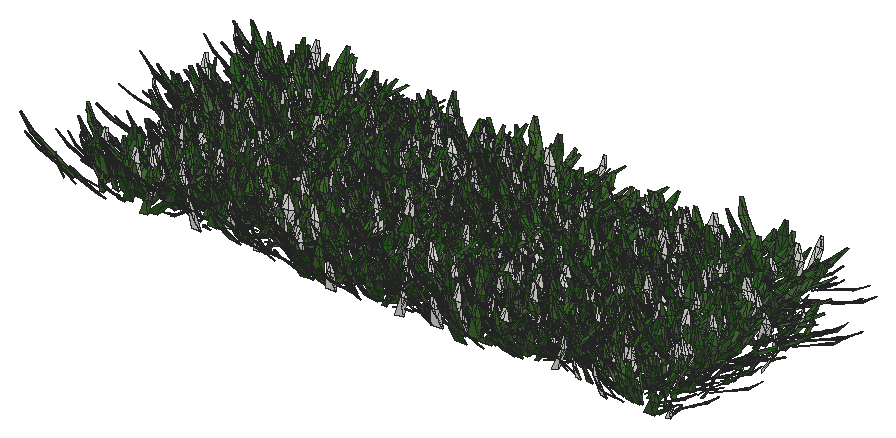
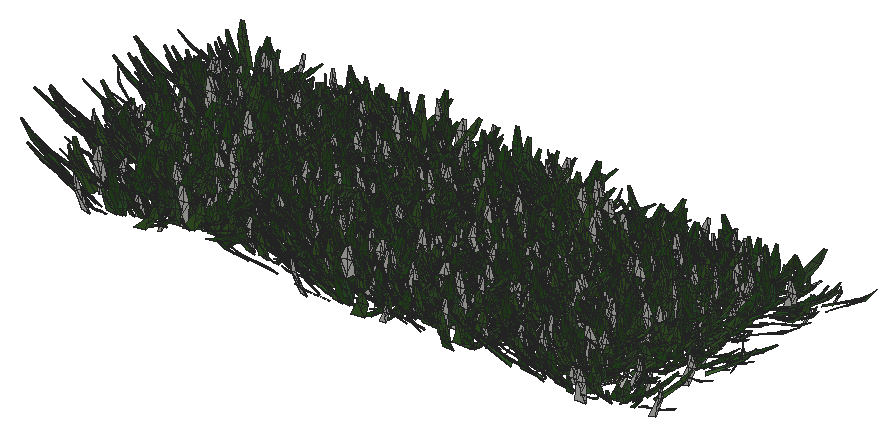
# SketchUp Ruby script. Lengths in inches.
U = 1.inch
M = Sketchup.active_model
def pt(a) = Geom::Point3d.new(a.map { |v| v * U })
def face(e, loops, mat)
  f = e.add_face(loops[0].map { |a| pt(a) })
  loops[1..].each { |l| e.add_face(l.map { |a| pt(a) }).erase! }
  f.material = f.back_material = mat if mat
  f
end
# faces: each face lists its corners as indices into pts; further lists are holes
def faces(e, pts, list, mat = nil) = list.each { |f| face(e, (f[0].is_a?(Array) ? f : [f]).map { |l| l.map { |i| pts[i] } }, mat) }
# xy, xz, yz: faces in a plane at the given z, y or x. An outline is a flat list of corners, or four numbers for a rectangle; further outlines are holes
def ring(l) = l.size == 4 ? [[l[0], l[1]], [l[2], l[1]], [l[2], l[3]], [l[0], l[3]]] : l.each_slice(2).to_a
def flat(e, list, mat, &to3) = list.each { |f| face(e, (f[0].is_a?(Array) ? f : [f]).map { |l| ring(l).map { |u, v| to3.(u, v) } }, mat) }
def xy(e, z, list, mat = nil) = flat(e, list, mat) { |x, y| [x, y, z] }
def xz(e, y, list, mat = nil) = flat(e, list, mat) { |x, z| [x, y, z] }
def yz(e, x, list, mat = nil) = flat(e, list, mat) { |y, z| [x, y, z] }
def lines(e, pts, list) = list.each { |a, b| e.add_line(pt(pts[a]), pt(pts[b])) }
# prism: a flat outline (further loops are holes) pulled along v
def prism(e, loops, v, mat = nil)
  f = face(e, loops, mat); d = Geom::Vector3d.new(v.map { |x| x * U })
  f.pushpull(f.normal.samedirection?(d) ? d.length : -d.length)
end
def box(e, o, s, mat = nil) = prism(e, [[o, [o[0] + s[0], o[1], o[2]], [o[0] + s[0], o[1] + s[1], o[2]], [o[0], o[1] + s[1], o[2]]]], [0, 0, s[2]], mat)
def at(x, y, z, deg = 0) = Geom::Transformation.translation(pt([x, y, z])) * Geom::Transformation.rotation(ORIGIN, Z_AXIS, deg.degrees)
def axes(o, x, y, z) = Geom::Transformation.new([*x, 0, *y, 0, *z, 0, *pt(o).to_a, 1])
def part(name) = M.definitions.add(name)
# library, detail: a bought-in or finely detailed component or shape, given as its bounding box
def library(name, o, s) = part(name).tap { |d| box(d.entities, o, s) }
def detail(e, o, s) = box(e.add_group.entities, o, s)
def put(e, d, t, mat = nil) = e.add_instance(d, t).tap { |i| i.material = mat if mat }
def group(e, t, mat = nil) = e.add_group.tap { |g| g.transformation = t; g.material = mat if mat }.entities
root = M.entities
M.materials.add("Material82").color = [68, 110, 58]
M.materials.add("Material83").color = [48, 90, 38]
M.materials.add("Material84").color = [68, 110, 48]
M.materials.add("Material85").color = [48, 90, 48]
M.materials.add("Material86").color = [58, 110, 58]
M.materials.add("Material87").color = [58, 90, 38]
M.materials.add("Material88").color = [68, 100, 58]
M.materials.add("Material89").color = [48, 100, 38]
c1 = part("grass00")
p = [[-0.6875,0.15,0],[-0.56,0.08,5.52],[-0.04,0.03,2.76],[0.48,-0.02,0],[0.35,-0.02,5.52],[-0.1,-0.14,5.52],
  [-0.12,0.65,8.37],[-0.42,0.65,8.37]]
faces(c1.entities,p,[[0,1,2,3],[3,2,4],[1,5,2],[5,4,2],[1,6,5],[4,5,6],[7,6,1]])
c2 = part("Group16\#1")
put(c2.entities,c1,axes([1.44,-0.61,-0.01],[0.05352,0.12609,0],[-0.10704,0.04543,0.07239],[0.06664,-0.02828,0.11628]),"Material85")
put(c2.entities,c1,axes([0.76,-0.15,-0.01],[0.04676,0.24062,0],[-0.23162,0.04501,0.06642],[0.0652,-0.01267,0.23595]),"Material82")
put(c2.entities,c1,axes([0.79,0.01,-0.01],[-0.00606,0.34651,0],[-0.34381,-0.00602,0.0432],[0.04319,0.00076,0.34386]))
put(c2.entities,c1,axes([1,0.23,-0.01],[-0.07192,0.31144,0],[-0.28722,-0.06632,0.1236],[0.12043,0.02781,0.29478]),"Material84")
put(c2.entities,c1,axes([1.66,0.77,-0.01],[-0.13828,0.29651,0],[-0.21551,-0.1005,0.22471],[0.20365,0.09498,0.23779]),"Material89")
put(c2.entities,c1,axes([0.6875,0.52,-0.01],[-0.18126,0.24051,0],[-0.22746,-0.17142,0.09788],[0.07817,0.05891,0.28481]),"Material84")
put(c2.entities,c1,axes([0.68,0.78,-0.01],[-0.215,0.18688,0],[-0.12385,-0.14248,0.21334],[0.13995,0.16101,0.18878]),"Material82")
put(c2.entities,c1,axes([0.56,1,-0.01],[-0.13756,0.07624,0],[-0.06159,-0.11112,0.0927],[0.04494,0.08108,0.12705]),"Material84")
put(c2.entities,c1,axes([0.2,0.64,-0.01],[-0.23729,0.07254,0],[-0.05711,-0.18681,0.153],[0.04473,0.14632,0.19535]),"Material89")
put(c2.entities,c1,axes([0.0625,0.72,-0.01],[-0.28874,0.02525,0],[-0.02179,-0.24916,0.14647],[0.01276,0.14591,0.25012]),"Material82")
put(c2.entities,c1,axes([-0.08,0.62,-0.01],[-0.34089,-0.04187,0],[0.03255,-0.26504,0.216],[-0.02633,0.21439,0.26703]),"Material89")
put(c2.entities,c1,axes([-0.34,0.98,-0.01],[-0.14314,-0.0493,0],[0.04397,-0.12769,0.06843],[-0.02228,0.0647,0.13505]),"Material89")
put(c2.entities,c1,axes([-0.87,1.45,-0.01],[-0.23488,-0.14114,0],[0.13761,-0.22901,0.06087],[-0.03135,0.05217,0.26717]))
put(c2.entities,c1,axes([-0.72,0.77,-0.01],[-0.14208,-0.13251,0],[0.07209,-0.0773,0.16301],[-0.11118,0.11922,0.1057]),"Material89")
put(c2.entities,c1,axes([-0.62,0.43,-0.01],[-0.14845,-0.21203,0],[0.18654,-0.13061,0.12304],[-0.10079,0.07057,0.22772]),"Material82")
put(c2.entities,c1,axes([-0.68,0.29,-0.01],[-0.13639,-0.32136,0],[0.31723,-0.13464,0.05579],[-0.05136,0.0218,0.34462]),"Material83")
put(c2.entities,c1,axes([-0.64,0.125,-0.01],[-0.0458,-0.23569,0],[0.22124,-0.043,0.08276],[-0.08124,0.01579,0.22538]),"Material86")
put(c2.entities,c1,axes([-1.6,-0.03,-0.01],[0.00576,-0.32897,0],[0.27526,0.00482,0.18018],[-0.18015,-0.00315,0.2753]),"Material84")
put(c2.entities,c1,axes([-1.36,-0.31,-0.01],[0.05718,-0.24765,0],[0.18172,0.04196,0.17267],[-0.16825,-0.03885,0.1865]),"Material89")
put(c2.entities,c1,axes([-1.54,-0.72,-0.01],[0.06537,-0.14017,0],[0.13555,0.06321,0.03939],[-0.0357,-0.01665,0.14956]))
put(c2.entities,c1,axes([-1.19,-0.9,-0.01],[0.09597,-0.12735,0],[0.11214,0.08451,0.07557],[-0.06035,-0.04548,0.14042]),"Material88")
put(c2.entities,c1,axes([-0.47,-0.54,-0.01],[0.11588,-0.10072,0],[0.0618,0.0711,0.12124],[-0.07953,-0.0915,0.0942]))
put(c2.entities,c1,axes([-0.47,-0.84,-0.01],[0.11927,-0.0661,0],[0.06603,0.11913,0.00646],[-0.00313,-0.00565,0.13621]),"Material84")
put(c2.entities,c1,axes([-0.38,-1.24,-0.01],[0.28037,-0.08571,0],[0.0618,0.20215,0.20315],[-0.05939,-0.19428,0.21139]),"Material88")
put(c2.entities,c1,axes([-0.06,-0.66,-0.01],[0.22719,-0.01987,0],[0.01247,0.14255,0.17758],[-0.01547,-0.17691,0.1431]),"Material87")
put(c2.entities,c1,axes([0.11,-0.89,-0.01],[0.14882,0.01828,0],[-0.01058,0.08611,0.12229],[0.01491,-0.12138,0.08676]),"Material85")
put(c2.entities,c1,axes([0.25,-0.72,-0.01],[0.20481,0.07053,0],[-0.06206,0.18022,0.10291],[0.03351,-0.0973,0.1906]),"Material85")
put(c2.entities,c1,axes([0.85,-1.42,-0.01],[0.16481,0.09904,0],[-0.09472,0.15762,0.05616],[0.02893,-0.04814,0.18389]),"Material84")
put(c2.entities,c1,axes([1.01,-1.09,-0.01],[0.21858,0.20385,0],[-0.17495,0.1876,0.15339],[0.10462,-0.11218,0.25652]),"Material89")
put(c2.entities,c1,axes([1.01,-0.71,-0.01],[0.08733,0.12473,0],[-0.06445,0.04512,0.13037],[0.1068,-0.07477,0.07867]),"Material85")
c3 = part("Group15\#1")
put(c3.entities,c2,at(0,0,0))
c4 = part("3darcstudiotree_grass00\#1")
put(c4.entities,c3,at(0,0,0))
put(root,c4,axes([1821.52,342.86,-34.17],[3.14963,-1.20842,0],[2.29792,0.93151,-0.01443],[0.07601,0.03081,1.86565]))
put(root,c4,axes([1822.68,356.8,-34.17],[-4.00454,-0.52801,0],[1.05814,-1.24816,-0.00172],[0.00311,-0.00367,1.42531]))
put(root,c4,axes([1822.78,343.67,-34.17],[-1.0046,-1.54951,0],[3.94346,-0.39764,-0.04783],[0.24428,-0.02463,1.6084]))
put(root,c4,axes([1821.28,366.74,-34.17],[2.75664,0.78459,0],[-2.60411,1.42301,-0.01696],[-0.0547,0.02989,1.8379]))
put(root,c4,axes([1821.49,355.92,-34.17],[1.57656,1.15501,0],[-3.7913,0.80487,-0.00648],[-0.02974,0.00631,1.68262]))
put(root,c4,axes([1823.79,345.66,-34.17],[-0.37683,-1.42813,0],[4.6236,-0.18974,-0.00351],[0.01488,-0.00061,1.48465]))
put(root,c4,axes([1822,340.73,-34.17],[4.54007,0.12562,0],[-0.30482,1.71344,-0.05051],[-0.02069,0.11631,1.91076]))
put(root,c4,axes([1823.4,350.05,-34.17],[1.62707,-1.18617,0],[3.8873,0.82932,-0.03985],[0.15889,0.0339,1.5017]))
put(root,c4,axes([1822.96,359.32,-34.17],[4.17569,0.70475,0],[-1.86329,1.71705,-0.06274],[-0.13365,0.12316,1.92197]))
put(root,c4,axes([1825.36,351.61,-34.17],[-3.80347,-0.79702,0],[1.88494,-1.39901,-0.03648],[0.10192,-0.07565,1.79293]))
put(root,c4,axes([1825.29,349.31,-34.17],[-2.17021,-1.46243,0],[2.84473,-0.65657,-0.0221],[0.14072,-0.03248,1.82262]))
put(root,c4,axes([1826.87,353.74,-34.17],[-2.18591,-1.17845,0],[3.11783,-0.89946,-0.02018],[0.10185,-0.02938,1.81061]))
put(root,c4,axes([1825.55,367.79,-34.17],[4.09864,-0.14348,0],[0.37168,1.65134,-0.01913],[0.00999,0.04439,1.86132]))
put(root,c4,axes([1826.16,355.56,-34.17],[-1.78032,1.61918,0],[-3.86174,-0.66038,-0.00354],[-0.01693,-0.0029,1.64409]))
put(root,c4,axes([1827.11,342.72,-34.17],[3.03313,0.50579,0],[-1.37798,1.28522,-0.04149],[-0.11611,0.10829,1.90578]))
put(root,c4,axes([1827.04,343.85,-34.17],[4.0409,0.57443,0],[-1.45336,1.59011,-0.05978],[-0.09434,0.10321,1.49495]))
put(root,c4,axes([1826.91,364.67,-34.17],[3.09052,1.16305,0],[-2.75216,1.13741,-0.00767],[-0.03246,0.01341,1.8325]))
put(root,c4,axes([1828.08,346.72,-34.17],[1.55138,-1.30688,0],[2.99369,0.55272,-0.04141],[0.29892,0.05519,1.97468]))
put(root,c4,axes([1827.93,360.0625,-34.17],[4.14328,-0.46419,0],[1.00154,1.39037,-0.02465],[0.03463,0.04808,1.41248]))
put(root,c4,axes([1828.45,358.2,-34.17],[-0.77153,1.33479,0],[-3.28421,-0.29525,-0.03421],[-0.24787,-0.02228,1.87625]))
put(root,c4,axes([1828.79,361.74,-34.17],[-1.91367,1.54924,0],[-4.25661,-0.81775,-0.00711],[-0.02422,-0.00465,1.34501]))
put(root,c4,axes([1829.4,366.36,-34.17],[3.43874,0.27286,0],[-0.6732,1.31953,-0.0192],[-0.02432,0.04768,1.64321]))
put(root,c4,axes([1830.92,343.8125,-34.17],[-4.1133,-0.05921,0],[0.15009,-1.6218,-0.04384],[0.00865,-0.09349,1.66887]))
put(root,c4,axes([1831.73,341.69,-34.17],[-3.5543,0.89209,0],[-1.79933,-1.11498,-0.04609],[-0.16829,-0.10428,1.7083]))
put(root,c4,axes([1832.4375,346.45,-34.17],[-2.34222,-1.01748,0],[3.28821,-1.17726,-0.05879],[0.21723,-0.07777,1.66118]))
put(root,c4,axes([1831.48,363.76,-34.17],[3.65348,-0.50094,0],[1.24961,1.41744,-0.02118],[0.04225,0.04793,1.73224]))
put(root,c4,axes([1832.65,359.43,-34.17],[-0.28709,-1.61704,0],[4.14071,-0.11434,-0.04142],[0.22933,-0.00633,1.72685]))
put(root,c4,axes([1831.33,366.19,-34.17],[1.27855,1.29921,0],[-4.02019,0.61532,-0.04732],[-0.19364,0.02964,1.41896]))
put(root,c4,axes([1831.85,350.0625,-34.17],[-1.96915,1.54328,0],[-4.06414,-0.80652,-0.00338],[-0.01619,-0.00321,1.82725]))
put(root,c4,axes([1833.39,349.04,-34.17],[-3.56597,0.54096,0],[-1.21057,-1.24113,-0.01112],[-0.02689,-0.02757,1.70172]))
put(root,c4,axes([1832.2,361.6,-34.17],[3.55843,0.77732,0],[-2.07504,1.47739,-0.02111],[-0.0608,0.04329,1.90804]))
put(root,c4,axes([1832.72,357.15,-34.17],[4.24476,0.21314,0],[-0.43337,1.34235,-0.04636],[-0.04216,0.1306,1.85211]))
put(root,c4,axes([1834.71,354.75,-34.17],[-3.8899,-0.78174,0],[2.11548,-1.63718,-0.02171],[0.04442,-0.03438,1.57387]))
put(root,c4,axes([1834.73,353.11,-34.17],[3.28347,0.12106,0],[-0.38901,1.64106,-0.04931],[-0.02254,0.09507,1.538]))
put(root,c4,axes([1837.52,354.72,-34.17],[-3.55041,0.9087,0],[-2.02381,-1.22981,-0.02727],[-0.0752,-0.0457,1.41127]))
put(root,c4,axes([1837.07,359.69,-34.17],[1.12356,1.5327,0],[-3.46853,0.39546,-0.04889],[-0.25471,0.02904,1.46761]))
put(root,c4,axes([1838.625,344.57,-34.17],[1.64327,-1.14246,0],[4.09949,0.91708,-0.03953],[0.17253,0.0386,1.77239]))
put(root,c4,axes([1837.41,342.6,-34.17],[0.41174,1.83159,0],[-3.96576,0.13865,-0.0152],[-0.08151,0.00285,1.60635]))
put(root,c4,axes([1839.55,348.04,-34.17],[0.23576,-1.73441,0],[4.70751,0.09952,-0.00697],[0.03732,0.00079,1.89407]))
put(root,c4,axes([1839.34,352.72,-34.17],[-3.49986,-0.57002,0],[1.44663,-1.38143,-0.04671],[0.11633,-0.11108,1.85324]))
put(root,c4,axes([1838.43,346.12,-34.17],[0.9145,1.75116,0],[-3.69114,0.2998,-0.03105],[-0.20233,0.01643,1.87912]))
put(root,c4,axes([1838.69,350.85,-34.17],[1.28043,1.73979,0],[-3.30316,0.37809,-0.03743],[-0.19576,0.02241,1.40382]))
put(root,c4,axes([1839.18,361.54,-34.17],[2.41483,0.92576,0],[-3.06998,1.24547,-0.04673],[-0.14351,0.05822,1.45453]))
put(root,c4,axes([1839.63,363.54,-34.17],[4.28624,-0.48224,0],[1.29741,1.79351,-0.04256],[0.05122,0.07081,1.55488]))
put(root,c4,axes([1839.96,365.39,-34.17],[0.63995,1.63517,0],[-3.50377,0.21327,-0.04631],[-0.28502,0.01735,1.65491]))
put(root,c4,axes([1840.43,357.61,-34.17],[4.08655,-0.74198,0],[1.4526,1.2443,-0.00355],[0.00912,0.00781,1.60125]))
put(root,c4,axes([1840.41,367.56,-34.17],[1.05791,1.29898,0],[-3.4169,0.4328,-0.04361],[-0.24845,0.03147,1.60948]))
put(root,c4,axes([1842.04,355.39,-34.17],[-0.24051,-1.38856,0],[3.98568,-0.10737,-0.04502],[0.19517,-0.00526,1.30109]))
put(root,c4,axes([1843.08,344.86,-34.17],[1.00632,-1.60929,0],[3.83281,0.37276,-0.00763],[0.0458,0.00445,1.82848]))
put(root,c4,axes([1843.68,350.2,-34.17],[-2.49579,-0.85332,0],[2.16334,-0.98408,-0.00893],[0.04692,-0.02134,1.98619]))
put(root,c4,axes([1843.63,364.02,-34.17],[2.15184,-1.02148,0],[3.44742,1.1295,-0.00974],[0.03611,0.01183,1.619]))
put(root,c4,axes([1844,352.47,-34.17],[-3.56783,-0.13568,0],[0.42403,-1.73414,-0.0118],[0.00459,-0.01877,1.34216]))
put(root,c4,axes([1843.34,357,-34.17],[4.22834,-0.67564,0],[1.61938,1.57623,-0.01357],[0.03127,0.03043,1.98263]))
put(root,c4,axes([1843.62,346.92,-34.17],[3.42011,0.99957,0],[-2.24279,1.19352,-0.03152],[-0.09807,0.05219,1.47514]))
put(root,c4,axes([1845.72,341.58,-34.17],[-0.92987,-1.7368,0],[3.78348,-0.31505,-0.00703],[0.03581,-0.00298,1.50812]))
put(root,c4,axes([1844.32,358.77,-34.17],[3.74003,-0.3626,0],[0.86697,1.39078,-0.02888],[0.04393,0.07047,1.73467]))
put(root,c4,axes([1845.92,349.15,-34.17],[-2.16285,-1.07783,0],[3.1191,-0.97346,-0.00813],[0.02825,-0.00882,1.32168]))
put(root,c4,axes([1844.33,366.05,-34.17],[2.54513,1.12368,0],[-2.54126,0.89522,-0.01423],[-0.07597,0.02676,1.82816]))
put(root,c4,axes([1845.34,362.52,-34.17],[-2.35271,1.42324,0],[-3.1761,-0.81658,-0.00573],[-0.02769,-0.00712,1.63969]))
put(root,c4,axes([1847.43,362.21,-34.17],[-2.99545,-1.01525,0],[2.44315,-1.12112,-0.00129],[0.00439,-0.00201,1.46122]))
put(root,c4,axes([1847.8,340.5,-34.17],[-4.11359,0.33172,0],[-0.73599,-1.4195,-0.0347],[-0.04072,-0.07853,1.61275]))
put(root,c4,axes([1849.05,355.09,-34.17],[-1.26006,-1.32624,0],[4.43512,-0.65537,-0.00645],[0.02239,-0.00331,1.31612]))
put(root,c4,axes([1847.46,347.21,-34.17],[0.26665,1.72733,0],[-3.78087,0.09078,-0.02381],[-0.14887,0.00357,1.77807]))
put(root,c4,axes([1848.7,356.875,-34.17],[0.22416,-1.4452,0],[4.13727,0.09981,-0.05271],[0.23324,0.00563,1.37729]))
put(root,c4,axes([1848.47,341.31,-34.17],[2.00643,-1.16557,0],[2.7626,0.73963,-0.03969],[0.18592,0.04978,1.41714]))
put(root,c4,axes([1849.375,353.65,-34.17],[-2.85144,-1.16634,0],[2.50888,-0.95396,-0.03577],[0.14723,-0.05598,1.49339]))
put(root,c4,axes([1848.15,350.85,-34.17],[1.02208,1.31259,0],[-4.10151,0.49672,-0.03259],[-0.17155,0.02078,1.77089]))
put(root,c4,axes([1848.15,364.71,-34.17],[2.93363,1.22701,0],[-2.56818,0.95498,-0.02839],[-0.14721,0.05474,1.88589]))
put(root,c4,axes([1850.06,360.3,-34.17],[-0.17296,-1.31916,0],[4.52056,-0.09218,-0.00424],[0.01978,-0.0004,1.58408]))
put(root,c4,axes([1851.19,348.625,-34.17],[-4.36692,-0.69342,0],[1.6396,-1.60594,-0.01703],[0.03175,-0.0311,1.64249]))
put(root,c4,axes([1851.2,365.94,-34.17],[-4.04807,0.23611,0],[-0.60438,-1.61163,-0.04443],[-0.03837,-0.10233,1.82802]))
put(root,c4,axes([1849.74,344.16,-34.17],[3.28108,0.9921,0],[-2.06723,1.06332,-0.03117],[-0.09708,0.04994,1.30357]))
put(root,c4,axes([1853.22,360.25,-34.17],[-3.17197,-0.90891,0],[2.49685,-1.35522,-0.03763],[0.13517,-0.07337,1.94544]))
put(root,c4,axes([1853.55,351.03,-34.17],[-3.35579,-1.19548,0],[2.90415,-1.2679,-0.0585],[0.2305,-0.10063,1.90866]))
put(root,c4,axes([1853.41,368.26,-34.17],[1.68348,-1.42,0],[3.90393,0.71983,-0.01397],[0.0682,0.01258,1.74087]))
put(root,c4,axes([1852.96,358.17,-34.17],[-1.26035,1.30994,0],[-3.37363,-0.50484,-0.03389],[-0.19382,-0.029,1.65454]))
put(root,c4,axes([1854.15,340.4,-34.17],[-3.39608,-0.38473,0],[1.21289,-1.66516,-0.05258],[0.08123,-0.11153,1.84274]))
put(root,c4,axes([1854.58,347.85,-34.17],[-0.07574,-1.47303,0],[4.38332,-0.03505,-0.05384],[0.21677,-0.00173,1.32332]))
put(root,c4,axes([1854.56,352.84,-34.17],[-3.58969,-0.07657,0],[0.18796,-1.37056,-0.00522],[0.00152,-0.01105,1.40302]))
put(root,c4,axes([1854.63,364.52,-34.17],[-3.78052,0.58265,0],[-1.19847,-1.20943,-0.02866],[-0.07958,-0.08031,1.88291]))
put(root,c4,axes([1855.4,355.84,-34.17],[-3.3619,-0.88005,0],[2.60897,-1.55009,-0.03911],[0.08798,-0.05227,1.43856]))
put(root,c4,axes([1854.84,345.96,-34.17],[-0.00326,-1.3732,0],[3.39922,-0.00125,-0.0371],[0.2688,-0.0001,1.84609]))
put(root,c4,axes([1855.62,365.9,-34.17],[-2.81078,-0.75848,0],[2.18011,-1.25652,-0.01797],[0.04803,-0.02768,1.36964]))
put(root,c4,axes([1854.7,344.97,-34.17],[3.61578,-1.02121,0],[2.66994,1.47029,-0.04389],[0.14306,0.07878,1.92393]))
put(root,c4,axes([1855.75,342.71,-34.17],[3.76801,-0.42175,0],[1.14915,1.59678,-0.03157],[0.04846,0.06733,1.77323]))
put(root,c4,axes([1856.05,361.52,-34.17],[2.09185,1.03032,0],[-2.8732,0.90727,-0.01526],[-0.08429,0.02662,1.9517]))
put(root,c4,axes([1859.09,351.16,-34.17],[-1.37112,-1.31689,0],[3.73876,-0.60543,-0.04381],[0.2334,-0.0378,1.74465]))
put(root,c4,axes([1859.71,364.17,-34.17],[-0.8424,-1.2576,0],[4.34376,-0.45254,-0.01354],[0.07406,-0.00772,1.90468]))
put(root,c4,axes([1858.9,358.94,-34.17],[3.65327,1.04493,0],[-2.10749,1.14596,-0.01189],[-0.03901,0.02121,1.50367]))
put(root,c4,axes([1860.14,354.6,-34.17],[-2.51613,1.14478,0],[-2.79457,-0.95529,-0.04719],[-0.16752,-0.05727,1.30223]))
put(root,c4,axes([1859.1875,365.96,-34.17],[3.43468,1.02641,0],[-2.59272,1.34938,-0.0181],[-0.04577,0.02382,1.34745]))
put(root,c4,axes([1860.95,341.85,-34.17],[-4.19905,0.34301,0],[-0.96105,-1.82979,-0.05761],[-0.05651,-0.10759,1.71741]))
put(root,c4,axes([1860.14,362.37,-34.17],[3.21656,-1.06764,0],[2.25071,1.05463,-0.04982],[0.17505,0.08203,1.4295]))
put(root,c4,axes([1861.58,345.05,-34.17],[0.12061,-1.58998,0],[4.18389,0.04936,-0.01737],[0.08566,0.00101,1.54781]))
put(root,c4,axes([1862.15,356.91,-34.17],[-3.70247,-0.49757,0],[1.50858,-1.74588,-0.06303],[0.09341,-0.1081,1.61067]))
put(root,c4,axes([1861.14,347.21,-34.17],[-0.34365,1.56469,0],[-3.45908,-0.11816,-0.04948],[-0.26965,-0.00921,1.42361]))
put(root,c4,axes([1860.69,352.77,-34.17],[1.76415,1.1719,0],[-3.51067,0.82196,-0.05173],[-0.20066,0.04698,1.38038]))
put(root,c4,axes([1861.45,348.74,-34.17],[4.55756,-0.02191,0],[0.04205,1.36049,-0.04731],[0.00354,0.1146,1.58849]))
put(root,c4,axes([1865.59,363.75,-34.17],[-3.74528,-0.54225,0],[1.29092,-1.38673,-0.02574],[0.04375,-0.047,1.38465]))
put(root,c4,axes([1865.48,360.06,-34.17],[-3.91187,0.00169,0],[-0.00401,-1.44027,-0.04481],[-0.00031,-0.10997,1.70362]))
put(root,c4,axes([1866.67,348.83,-34.17],[-3.9934,-0.49353,0],[1.06998,-1.34652,-0.00157],[0.00241,-0.00304,1.37913]))
put(root,c4,axes([1866.61,340.58,-34.17],[-1.39646,-1.43145,0],[3.7454,-0.56828,-0.0371],[0.22587,-0.03427,1.96201]))
put(root,c4,axes([1865.52,365.71,-34.17],[2.25108,1.29367,0],[-3.07657,0.83262,-0.0512],[-0.2098,0.05678,1.38975]))
put(root,c4,axes([1866.21,357.38,-34.17],[-1.78787,1.37846,0],[-3.47115,-0.7002,-0.05082],[-0.20934,-0.04223,1.35221]))
put(root,c4,axes([1865.48,355.66,-34.17],[3.1901,1.34772,0],[-3.0794,1.13365,-0.04297],[-0.19725,0.07262,1.98261]))
put(root,c4,axes([1866.96,361.08,-34.17],[-3.49916,1.06741,0],[-2.60054,-1.32589,-0.05181],[-0.14447,-0.07366,1.45196]))
put(root,c4,axes([1867.16,353.76,-34.17],[-3.70101,0.79314,0],[-2.22235,-1.61286,-0.04664],[-0.10432,-0.07571,1.63424]))
put(root,c4,axes([1865.86,342.17,-34.17],[1.4538,1.50227,0],[-4.10712,0.61817,-0.00597],[-0.03083,0.00464,1.82255]))
put(root,c4,axes([1867.125,346.49,-34.17],[-1.85188,1.07885,0],[-3.29338,-0.87924,-0.00267],[-0.01201,-0.00321,1.62102]))
put(root,c4,axes([1867.86,350.35,-34.17],[2.80724,-1.17226,0],[3.04027,1.13235,-0.05261],[0.16943,0.06311,1.38839]))
put(root,c4,axes([1867.19,344.08,-34.17],[3.28196,0.81984,0],[-2.45781,1.53025,-0.01012],[-0.02495,0.01554,1.58691]))
put(root,c4,axes([1869.83,348.75,-34.17],[-0.83235,-1.28841,0],[3.31595,-0.33318,-0.03395],[0.19708,-0.0198,1.53644]))
put(root,c4,axes([1870.17,352.37,-34.17],[-0.43709,-1.41781,0],[4.63894,-0.22243,-0.04217],[0.16902,-0.0081,1.41426]))
put(root,c4,axes([1869.6,357.96,-34.17],[3.88367,-0.39615,0],[1.13822,1.73547,-0.04841],[0.06323,0.0964,1.77682]))
put(root,c4,axes([1871.05,342.02,-34.17],[-0.85576,-1.5606,0],[4.52661,-0.38605,-0.05631],[0.21879,-0.01866,1.37991]))
put(root,c4,axes([1871.31,355.05,-34.17],[-2.86852,-0.72551,0],[1.94813,-1.19796,-0.01822],[0.05809,-0.03572,1.59761]))
put(root,c4,axes([1871.07,345.8,-34.17],[-3.59941,0.74413,0],[-1.52837,-1.14979,-0.02232],[-0.06679,-0.05025,1.59039]))
put(root,c4,axes([1869.7,359.95,-34.17],[1.48622,1.27925,0],[-3.96463,0.71638,-0.00338],[-0.01448,0.00262,1.53978]))
put(root,c4,axes([1871.6875,363.74,-34.17],[1.63817,-1.67164,0],[3.7967,0.57868,-0.011],[0.05001,0.00762,1.48653]))
put(root,c4,axes([1872.13,340.65,-34.17],[-2.82588,-0.78458,0],[2.18733,-1.22531,-0.03828],[0.15336,-0.08591,1.98208]))
put(root,c4,axes([1873.13,345.03,-34.17],[-1.60743,-1.14355,0],[3.95374,-0.86436,-0.00731],[0.03731,-0.00816,1.97847]))
put(root,c4,axes([1873.16,361.95,-34.17],[-3.32772,0.28661,0],[-0.75668,-1.36642,-0.01018],[-0.01111,-0.02006,1.35975]))
put(root,c4,axes([1872.1875,350.23,-34.17],[3.98724,0.20884,0],[-0.61603,1.82924,-0.05242],[-0.03685,0.10943,1.87281]))
put(root,c4,axes([1873.1875,365.46,-34.17],[-0.30333,1.33059,0],[-3.40704,-0.1208,-0.0349],[-0.19211,-0.00681,1.41691]))
put(root,c4,axes([1876.4375,342.5625,-34.17],[-2.807,-0.90771,0],[2.30635,-1.10925,-0.04795],[0.15506,-0.07458,1.39039]))
put(root,c4,axes([1875.5,345.74,-34.17],[3.2807,-0.61041,0],[1.81668,1.51857,-0.02435],[0.05518,0.04613,1.69455]))
put(root,c4,axes([1876.68,360.95,-34.17],[-1.43959,-1.62411,0],[3.7168,-0.5124,-0.03865],[0.23963,-0.03303,1.9383]))
put(root,c4,axes([1877.375,363.94,-34.17],[-3.81782,0.15844,0],[-0.49654,-1.86087,-0.00853],[-0.00435,-0.0163,1.7318]))
put(root,c4,axes([1878.07,349.4,-34.17],[-3.12571,-0.7496,0],[2.43282,-1.57777,-0.06276],[0.13907,-0.09019,1.49667]))
put(root,c4,axes([1876.45,344.7,-34.17],[2.97603,0.7742,0],[-2.07464,1.24033,-0.03997],[-0.14341,0.08574,1.84008]))
put(root,c4,axes([1878.3,352.43,-34.17],[-2.31531,-0.95478,0],[2.79879,-1.05558,-0.03327],[0.10847,-0.04091,1.30962]))
put(root,c4,axes([1878.37,357.14,-34.17],[-3.94904,-0.28889,0],[0.74698,-1.58808,-0.00704],[0.00779,-0.01657,1.86241]))
put(root,c4,axes([1877.27,366.4375,-34.17],[-1.72673,1.11938,0],[-3.66172,-0.8785,-0.02284],[-0.09991,-0.02397,1.64481]))
put(root,c4,axes([1877.68,350.12,-34.17],[-0.65898,1.54379,0],[-3.85922,-0.25621,-0.04712],[-0.21087,-0.014,1.33133]))
put(root,c4,axes([1877.28,355.43,-34.17],[1.80555,1.12349,0],[-3.92794,0.98179,-0.01772],[-0.05919,0.0148,1.37883]))
put(root,c4,axes([1879.1,358.93,-34.17],[-2.45667,1.24552,0],[-3.48685,-1.06965,-0.01031],[-0.04097,-0.01257,1.66779]))
put(root,c4,axes([1880.63,350.98,-34.17],[-1.11481,1.68554,0],[-3.85911,-0.39697,-0.04083],[-0.25467,-0.0262,1.92702]))
put(root,c4,axes([1881.15,365.85,-34.17],[3.83562,-0.64652,0],[1.50566,1.38929,-0.01454],[0.02594,0.02394,1.30369]))
put(root,c4,axes([1881.99,363.77,-34.17],[-3.30618,0.81403,0],[-2.41899,-1.52802,-0.02972],[-0.07466,-0.04716,1.62371]))
put(root,c4,axes([1883.56,346.76,-34.17],[-3.64839,-0.0594,0],[0.18827,-1.79867,-0.05407],[0.01098,-0.10487,1.68402]))
put(root,c4,axes([1882.11,341.67,-34.17],[2.37064,0.94684,0],[-3.28047,1.27743,-0.04002],[-0.15051,0.05861,1.82631]))
put(root,c4,axes([1883.07,361.67,-34.17],[-3.05865,1.0781,0],[-2.78611,-1.22937,-0.02716],[-0.07662,-0.03381,1.32671]))
put(root,c4,axes([1884.19,359.27,-34.17],[-2.13062,-1.66467,0],[3.82642,-0.7617,-0.02075],[0.09652,-0.01921,1.67433]))
put(root,c4,axes([1884.14,348.76,-34.17],[-4.39804,-0.22301,0],[0.45888,-1.40747,-0.03967],[0.03344,-0.10258,1.78282]))
put(root,c4,axes([1883.5,368.15,-34.17],[2.97779,-1.31333,0],[2.93322,1.03437,-0.03435],[0.15944,0.05623,1.83666]))
put(root,c4,axes([1884.44,355.65,-34.17],[-3.86294,0.12208,0],[-0.37038,-1.82279,-0.02116],[-0.00872,-0.04291,1.79229]))
put(root,c4,axes([1884.51,357.86,-34.17],[4.62049,-0.36242,0],[0.91883,1.82189,-0.02703],[0.02558,0.05072,1.71263]))
put(root,c4,axes([1884.4,352.21,-34.17],[4.4065,0.29877,0],[-0.73465,1.68517,-0.00744],[-0.00712,0.01634,1.83611]))
put(root,c4,axes([1884.48,344.4,-34.17],[2.92133,1.34194,0],[-2.9494,0.99861,-0.03135],[-0.14252,0.04825,1.74596]))
put(root,c4,axes([1886.25,359.25,-34.17],[-4.37191,-0.09188,0],[0.22077,-1.63377,-0.04256],[0.01218,-0.09013,1.67228]))
put(root,c4,axes([1886.88,351,-34.17],[-0.6545,-1.64207,0],[4.59681,-0.28496,-0.0381],[0.20859,-0.01293,1.93318]))
put(root,c4,axes([1886.27,345.98,-34.17],[3.15887,-0.80876,0],[1.92191,1.16751,-0.02789],[0.09845,0.05981,1.71527]))
put(root,c4,axes([1887.1,347.97,-34.17],[-3.60106,0.31713,0],[-0.9107,-1.60836,-0.00123],[-0.0017,-0.003,1.99006]))
put(root,c4,axes([1886.98,344.0625,-34.17],[1.90217,1.207,0],[-3.00756,0.73717,-0.00184],[-0.00944,0.00231,1.60144]))
put(root,c4,axes([1887.89,340.08,-34.17],[-1.8058,1.22943,0],[-3.0103,-0.68768,-0.02138],[-0.11593,-0.02648,1.63406]))
put(root,c4,axes([1887.88,357.88,-34.17],[-1.11998,1.52641,0],[-4.36702,-0.49835,-0.06381],[-0.30025,-0.03426,1.66913]))
